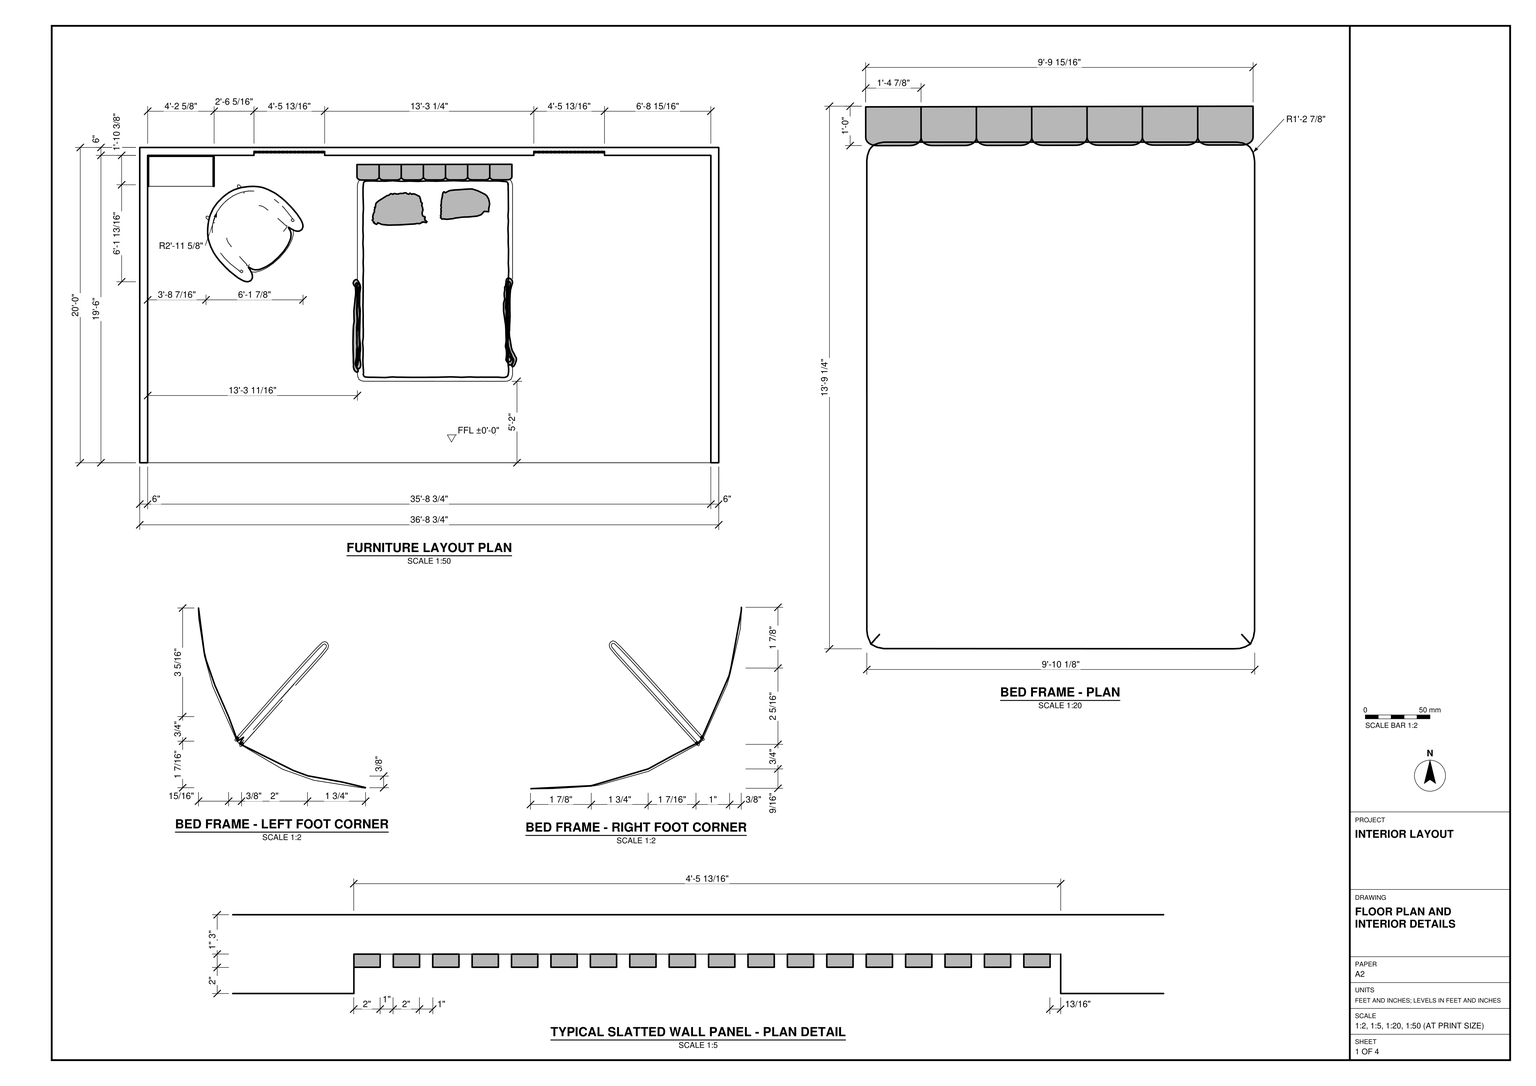
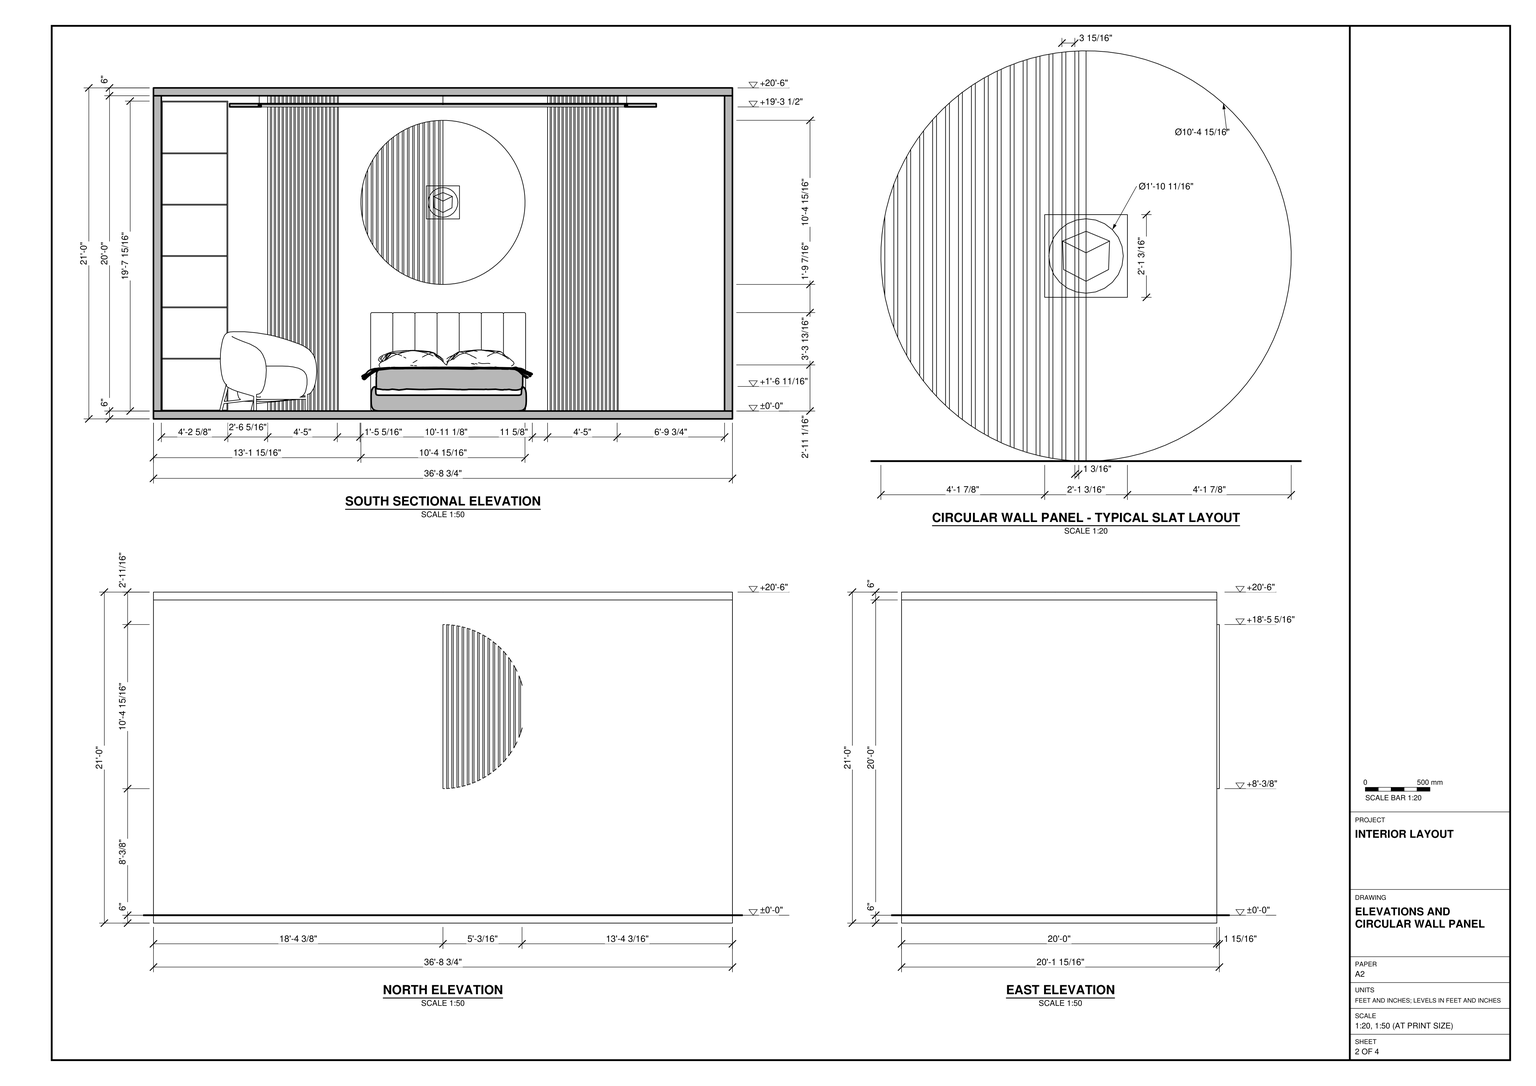
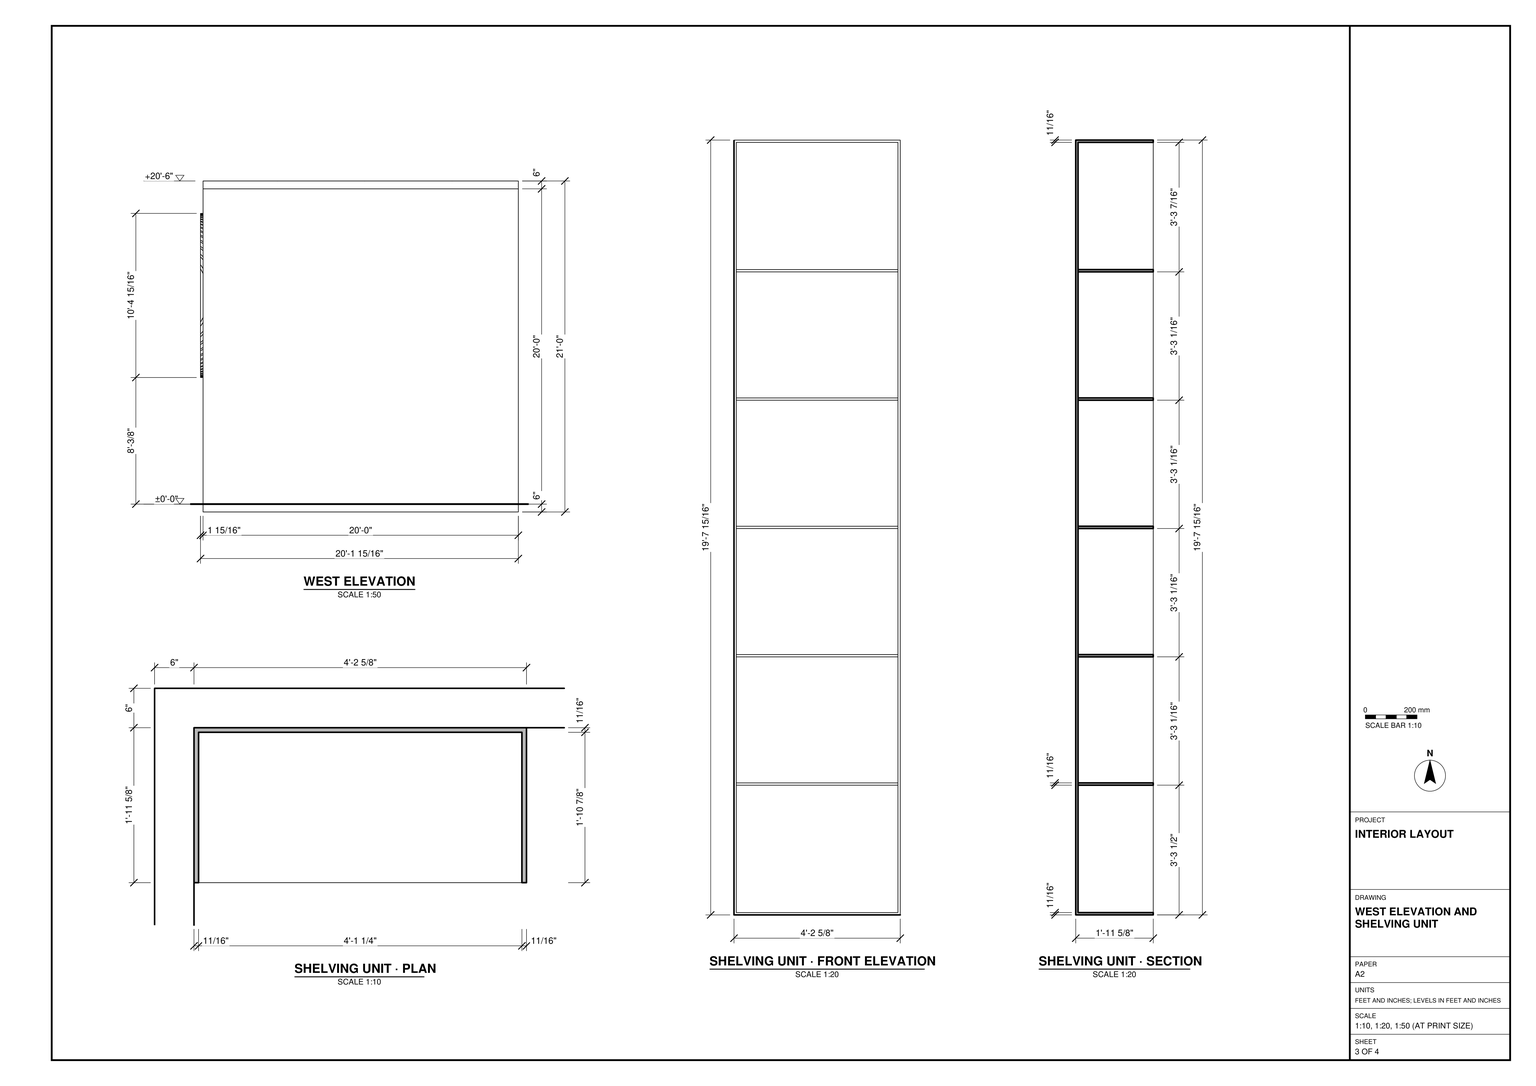
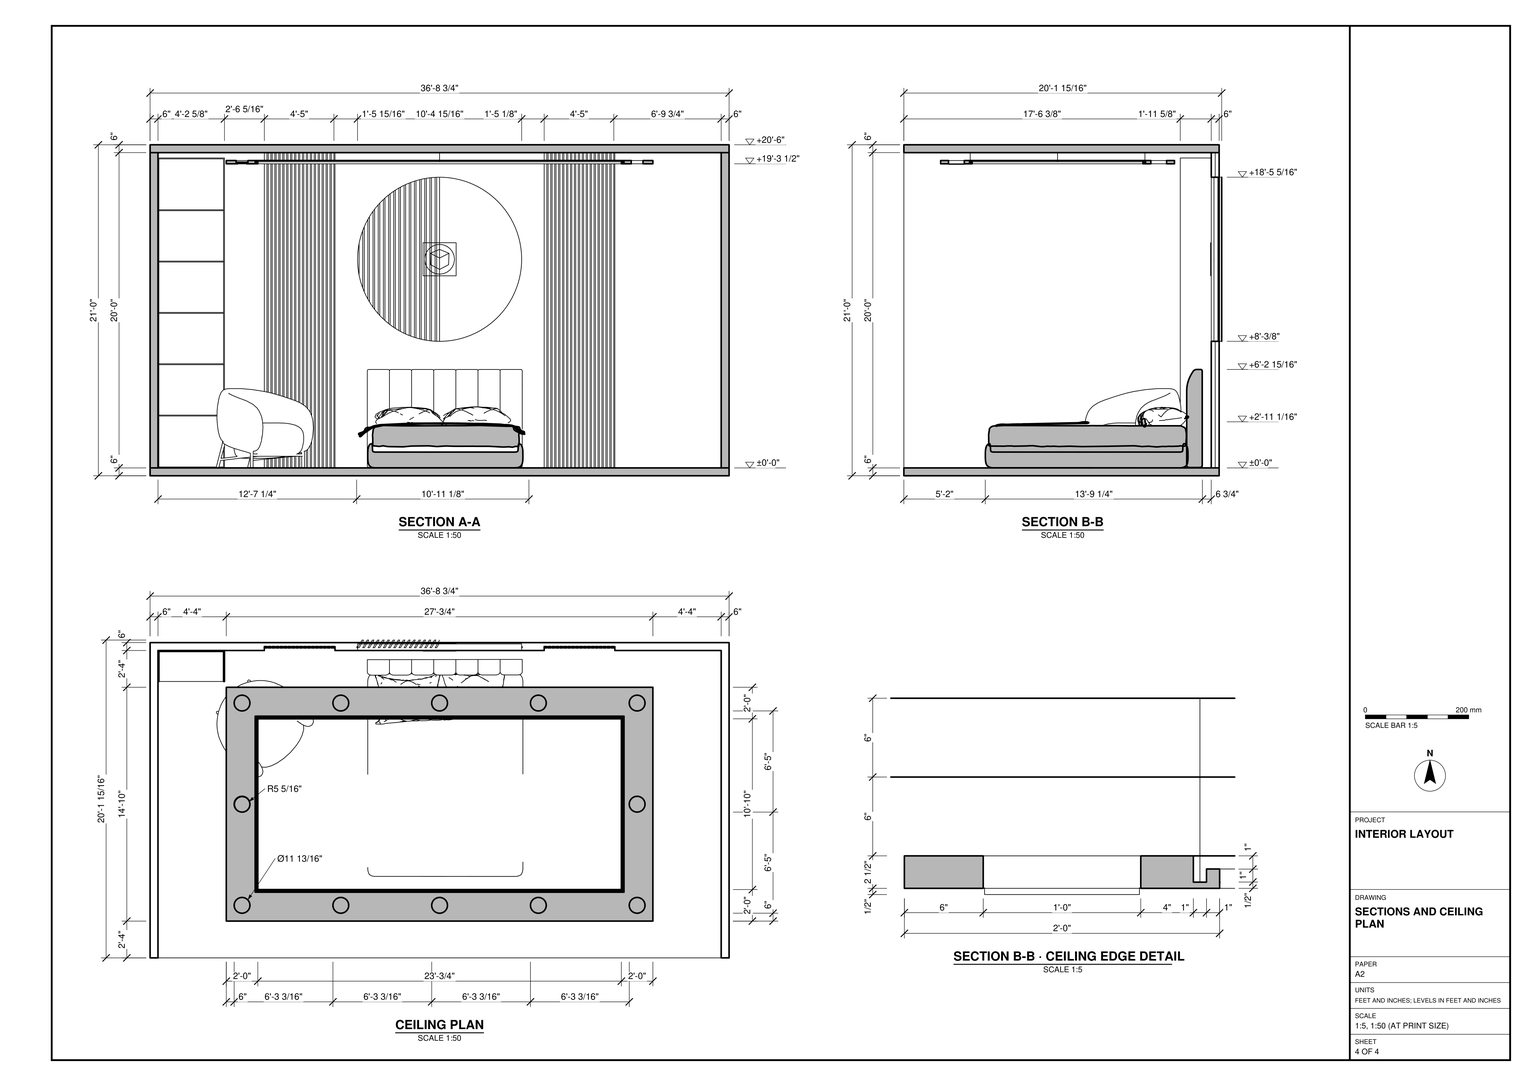
Build the bedroom interior in SketchUp from task_files/diagram_01.pdf. Work in feet and inches. Set the finished floor level to ±0'-0". The overall model, including the projecting wall detail, is 36'-8 3/4" wide, 20'-1 15/16" deep and 21'-0" high. Form the north wall and both side walls at 6" thick, leaving the south side open as drawn. Include the 6" floor and ceiling slabs, with a clear height of 20'-0" between them.

Place the bed with its segmented headboard against the north wall and its foot facing the open side. Follow the bed-frame plan for the rounded foot corners, and use the sectional elevation to set the mattress and headboard heights. Above the bed, model the circular wall panel with vertical slats on its left half and a plain field on its right. Flank the bed with the two tall rectangular slatted panels, following the spacing in the plan detail. Fit the tall open shelving unit into the northwest corner and place the armchair in front of it, angled as shown in the furniture layout.

Keep the walls and slabs separate, and make each furniture or joinery piece a separate group or component. Use components for repeated parts such as slats. Decor and loose items may be any suitable library components. Save one SketchUp model as output_files/bedroom_with_slatted_wall_panels_and_built_in_shelving.skp.

# SketchUp Ruby script. Lengths in inches.
U = 1.inch
M = Sketchup.active_model
def pt(a) = Geom::Point3d.new(a.map { |v| v * U })
def face(e, loops, mat)
  f = e.add_face(loops[0].map { |a| pt(a) })
  loops[1..].each { |l| e.add_face(l.map { |a| pt(a) }).erase! }
  f.material = f.back_material = mat if mat
  f
end
# faces: each face lists its corners as indices into pts; further lists are holes
def faces(e, pts, list, mat = nil) = list.each { |f| face(e, (f[0].is_a?(Array) ? f : [f]).map { |l| l.map { |i| pts[i] } }, mat) }
# xy, xz, yz: faces in a plane at the given z, y or x. An outline is a flat list of corners, or four numbers for a rectangle; further outlines are holes
def ring(l) = l.size == 4 ? [[l[0], l[1]], [l[2], l[1]], [l[2], l[3]], [l[0], l[3]]] : l.each_slice(2).to_a
def flat(e, list, mat, &to3) = list.each { |f| face(e, (f[0].is_a?(Array) ? f : [f]).map { |l| ring(l).map { |u, v| to3.(u, v) } }, mat) }
def xy(e, z, list, mat = nil) = flat(e, list, mat) { |x, y| [x, y, z] }
def xz(e, y, list, mat = nil) = flat(e, list, mat) { |x, z| [x, y, z] }
def yz(e, x, list, mat = nil) = flat(e, list, mat) { |y, z| [x, y, z] }
def lines(e, pts, list) = list.each { |a, b| e.add_line(pt(pts[a]), pt(pts[b])) }
# prism: a flat outline (further loops are holes) pulled along v
def prism(e, loops, v, mat = nil)
  f = face(e, loops, mat); d = Geom::Vector3d.new(v.map { |x| x * U })
  f.pushpull(f.normal.samedirection?(d) ? d.length : -d.length)
end
def box(e, o, s, mat = nil) = prism(e, [[o, [o[0] + s[0], o[1], o[2]], [o[0] + s[0], o[1] + s[1], o[2]], [o[0], o[1] + s[1], o[2]]]], [0, 0, s[2]], mat)
def at(x, y, z, deg = 0) = Geom::Transformation.translation(pt([x, y, z])) * Geom::Transformation.rotation(ORIGIN, Z_AXIS, deg.degrees)
def axes(o, x, y, z) = Geom::Transformation.new([*x, 0, *y, 0, *z, 0, *pt(o).to_a, 1])
def part(name) = M.definitions.add(name)
# library, detail: a bought-in or finely detailed component or shape, given as its bounding box
def library(name, o, s) = part(name).tap { |d| box(d.entities, o, s) }
def detail(e, o, s) = box(e.add_group.entities, o, s)
def put(e, d, t, mat = nil) = e.add_instance(d, t).tap { |i| i.material = mat if mat }
def group(e, t, mat = nil) = e.add_group.tap { |g| g.transformation = t; g.material = mat if mat }.entities
root = M.entities
M.materials.add("WALL").color = [163, 159, 147]
M.materials.add("Wood 009 27.06cm").color = [255, 255, 255]
c1 = part("Group66\#1")
p = [[0,0,0],[0,0,-7.89],[-3.85,0,-7.89],[25.04,-0.51,0],[-25.04,-0.51,0],[25.04,0.51,0],
  [25.04,0,0],[-25.04,0.51,0],[3.85,0,-7.89],[-25.04,0,0],[0,0,-12.77]]
lines(c1.entities,p,[[0,1],[1,2],[3,4],[5,6],[7,5],[1,8],[9,0],[0,6],[8,10],[4,9],[6,3],[2,10],
  [9,7]])
c2 = part("shelves")
put(c2.entities,c1,at(0,0,0))
c3 = library("BED 3",[-244.73,-59.6875,196.6875],[91.01,69.4,39.64])
c4 = library("Armchair 287 004",[-17.02,-16.23,-0.09],[34.04,32.42,30.2])
c5 = part("Group5\#1")
xy(c5.entities,0,[[-26.65,-23.47,-27.78,-20.53,-27.84,-20.33,-27.84,20.25,-27.32,21.79,-26.65,23.42]])
xy(c5.entities,5.875,[[-30.05,-12.08,-30.05,12.03,-30.37,10.43,-30.9,6.55,-31.19,2.63,-31.23,-1.29,-31.03,-5.21,-30.58,-9.11]])
p = [[-30.05,12.03,5.875],[-30.05,-12.08,5.875],[-29.89,-12.98,5.6],[-28.95,-16.79,3.98],[-27.78,-20.53,1.95],[-26.65,-23.47,0],
  [-26.65,23.42,0],[-27.32,21.79,1.15],[-28.57,18.07,3.33],[-29.59,14.28,5.09],[-31.03,-5.21,5.52],[-31.23,-1.29,5.875],
  [-31.19,2.63,5.8],[-30.9,6.55,5.3],[-30.37,10.43,4.375],[-29.59,14.28,3.03],[-28.57,18.07,1.27],[-27.84,20.25,0],
  [-27.84,-20.33,0],[-28.95,-16.79,1.92],[-29.89,-12.98,3.54],[-30.58,-9.11,4.74]]
faces(c5.entities,p,[[0,1,2,3,4,5,6,7,8,9],[10,11,12,13,14,15,16,17,18,19,20,21]])
c6 = part("Group6\#1")
xy(c6.entities,0,[[-22.72,-31.5,-22.89,-31.23,-23.9,-29.33,-23.9,29.35,-22.72,31.46]])
xy(c6.entities,5.875,[[-26.11,-24.78,-26.11,24.76,-27.3,21.85,-27.3,-21.79,-26.375,-24.2]])
p = [[-26.11,24.76,5.875],[-26.11,-24.78,5.875],[-24.74,-27.77,3.51],[-22.89,-31.23,0.29],[-22.72,-31.5,0],[-22.72,31.46,0],
  [-24.13,28.96,2.44],[-25.84,25.43,5.4],[-27.3,-21.79,5.875],[-27.3,21.85,5.875],[-25.84,25.43,3.35],[-24.13,28.96,0.39],
  [-23.9,29.35,0],[-23.9,-29.33,0],[-24.74,-27.77,1.45],[-26.375,-24.2,4.28]]
faces(c6.entities,p,[[0,1,2,3,4,5,6,7],[8,9,10,11,12,13,14,15]])
c7 = part("Group7\#1")
xy(c7.entities,0,[[-18.78,-37.4375,-19.97,-35.77,-19.97,35.8,-18.78,37.39]])
xy(c7.entities,5.875,[[-22.17,-32.38,-22.17,32.42,-22.2,32.38,-23.36,30.32,-23.36,-30.35,-22.89,-31.23]])
p = [[-18.78,-37.4375,0],[-18.78,37.39,0],[-20.06,35.67,2.22],[-22.17,32.42,5.875],[-22.17,-32.38,5.875],[-20.82,-34.57,3.53],
  [-23.36,-30.35,5.875],[-23.36,30.32,5.875],[-22.2,32.38,3.87],[-20.06,35.67,0.16],[-19.97,35.8,0],[-19.97,-35.77,0],
  [-20.82,-34.57,1.48],[-22.89,-31.23,5.06]]
faces(c7.entities,p,[[0,1,2,3,4,5],[6,7,8,9,10,11,12,13]])
c8 = part("Group8\#1")
xy(c8.entities,0,[[-14.84,-42.16,-16.03,-40.87,-16.03,40.82,-15.18,41.82,-14.84,42.17]])
xy(c8.entities,5.875,[[-18.23,-38.15,-18.23,38.125,-19.42,36.53,-19.42,-36.53,-18.55,-37.77]])
p = [[-14.84,-42.16,0],[-14.84,42.17,0],[-15.18,41.82,0.59],[-17.72,38.82,4.98],[-18.23,38.125,5.875],[-18.23,-38.15,5.875],
  [-16.08,-40.82,2.14],[-19.42,-36.53,5.875],[-19.42,36.53,5.875],[-17.72,38.82,2.93],[-16.03,40.82,0],[-16.03,-40.87,0],
  [-16.08,-40.82,0.08],[-18.55,-37.77,4.36]]
faces(c8.entities,p,[[0,1,2,3,4,5,6],[7,8,9,10,11,12,13]])
c9 = part("Group9\#1")
xy(c9.entities,0,[[-10.9,-46.125,-12.09,-44.98,-12.09,44.99,-10.9,46.08]])
xy(c9.entities,5.875,[[-14.3,-42.76,-14.3,42.74,-15.18,41.82,-15.48,41.46,-15.48,-41.46]])
p = [[-14.3,42.74,5.875],[-14.3,-42.76,5.875],[-13.42,-43.71,4.36],[-10.9,-46.125,0],[-10.9,46.08,0],[-12.47,44.65,2.7],
  [-15.48,-41.46,5.875],[-15.48,41.46,5.875],[-15.18,41.82,5.36],[-12.47,44.65,0.65],[-12.09,44.99,0],[-12.09,-44.98,0],
  [-13.42,-43.71,2.3]]
faces(c9.entities,p,[[0,1,2,3,4,5],[6,7,8,9,10,11,12]])
c10 = part("Group10\#1")
xy(c10.entities,0,[[-6.97,-49.43,-7.59,-48.96,-8.15,-48.49,-8.15,48.46,-6.97,49.42]])
xy(c10.entities,5.875,[[-10.36,-46.62,-10.36,46.59,-11.55,45.49,-11.55,-45.51,-10.59,-46.43]])
p = [[-6.97,-49.43,0],[-6.97,49.42,0],[-9.58,47.31,4.52],[-10.36,46.59,5.875],[-10.36,-46.62,5.875],[-7.59,-48.96,1.08],
  [-8.15,48.46,0],[-8.15,-48.49,0],[-10.59,-46.43,4.22],[-11.55,-45.51,5.875],[-11.55,45.49,5.875],[-9.58,47.31,2.46]]
faces(c10.entities,p,[[0,1,2,3,4,5],[6,7,8,9,10,11]])
c11 = part("Group11\#1")
xy(c11.entities,0,[[-3.03,-52.22,-4.22,-51.45,-4.22,51.41,-3.32,52.05,-3.03,52.23]])
xy(c11.entities,5.875,[[-6.42,-49.83,-6.42,49.85,-6.53,49.77,-7.61,48.9,-7.61,-48.95,-7.59,-48.96]])
p = [[-3.03,-52.22,0],[-3.03,52.23,0],[-3.32,52.05,0.51],[-6.42,49.85,5.875],[-6.42,-49.83,5.875],[-4.44,-51.3,2.45],
  [-4.22,51.41,0],[-4.22,-51.45,0],[-4.44,-51.3,0.39],[-7.59,-48.96,5.85],[-7.61,-48.95,5.875],[-7.61,48.9,5.875],
  [-6.53,49.77,4]]
faces(c11.entities,p,[[0,1,2,3,4,5],[6,7,8,9,10,11,12]])
c12 = part("Group12\#1")
xy(c12.entities,0,[[0.91,-54.6,-0.28,-53.93,-0.28,53.93,0.01,54.11,0.91,54.59]])
xy(c12.entities,5.875,[[-2.48,-52.57,-2.48,52.57,-3.32,52.05,-3.67,51.8,-3.67,-51.8]])
p = [[0.91,-54.6,0],[0.91,54.59,0],[0.01,54.11,1.55],[-2.48,52.57,5.875],[-2.48,-52.57,5.875],[-1.15,-53.44,3.57],
  [-3.67,-51.8,5.875],[-3.67,51.8,5.875],[-3.32,52.05,5.27],[-0.28,53.93,0],[-0.28,-53.93,0],[-1.15,-53.44,1.51]]
faces(c12.entities,p,[[0,1,2,3,4,5],[6,7,8,9,10,11]])
c13 = part("Group13\#1")
xy(c13.entities,0,[[4.85,-56.62,3.66,-56.04,3.66,56.05,4.85,56.6]])
xy(c13.entities,5.875,[[1.45,-54.91,1.45,54.89,0.27,54.25,0.27,-54.24]])
p = [[1.45,54.89,5.875],[1.45,-54.91,5.875],[2.27,-55.37,4.46],[4.85,-56.62,0],[4.85,56.6,0],[3.47,55.97,2.38],
  [3.66,56.05,0],[3.66,-56.04,0],[2.27,-55.37,2.41],[0.27,-54.24,5.875],[0.27,54.25,5.875],[3.47,55.97,0.32]]
faces(c13.entities,p,[[0,1,2,3,4,5],[6,7,8,9,10,11]])
c14 = part("Group14\#1")
xy(c14.entities,0,[[8.78,-58.3,7.6,-57.8125,7.6,57.8125,8.78,58.27]])
xy(c14.entities,5.875,[[5.39,-56.88,5.39,56.85,4.2,56.3,4.2,-56.31]])
p = [[8.78,-58.3,0],[8.78,58.27,0],[7.04,57.6,3.02],[5.39,56.85,5.875],[5.39,-56.88,5.875],[5.8,-57.08,5.16],
  [4.2,-56.31,5.875],[4.2,56.3,5.875],[7.04,57.6,0.96],[7.6,57.8125,0],[7.6,-57.8125,0],[5.8,-57.08,3.11]]
faces(c14.entities,p,[[0,1,2,3,4,5],[6,7,8,9,10,11]])
c15 = part("Group15\#1")
xy(c15.entities,0,[[12.72,-59.67,11.53,-59.27,11.53,59.27,12.72,59.64]])
xy(c15.entities,5.875,[[9.33,-58.52,9.33,58.48,8.14,58.02,8.14,-58.03]])
p = [[12.72,-59.67,0],[12.72,59.64,0],[10.71,59.01,3.49],[9.33,58.48,5.875],[9.33,-58.52,5.875],[9.43,-58.5625,5.69],
  [8.14,-58.03,5.875],[8.14,58.02,5.875],[10.71,59.01,1.43],[11.53,59.27,0],[11.53,-59.27,0],[9.43,-58.5625,3.63]]
faces(c15.entities,p,[[0,1,2,3,4,5],[6,7,8,9,10,11]])
c16 = part("Group16\#1")
xy(c16.entities,0,[[16.66,-60.76,15.47,-60.4375,15.47,60.43,16.66,60.72]])
xy(c16.entities,5.875,[[13.27,-59.85,13.27,59.81,12.08,59.4375,12.08,-59.45,13.15,-59.82]])
p = [[13.27,59.81,5.875],[13.27,-59.85,5.875],[16.66,-60.76,0],[16.66,60.72,0],[14.45,60.18,3.82],[12.08,-59.45,5.875],
  [12.08,59.4375,5.875],[14.45,60.18,1.76],[15.47,60.43,0],[15.47,-60.4375,0],[13.15,-59.82,4.01]]
faces(c16.entities,p,[[0,1,2,3,4],[5,6,7,8,9,10]])
c17 = part("Group17\#1")
xy(c17.entities,0,[[20.6,-61.57,19.41,-61.33,19.41,61.32,20.6,61.53]])
xy(c17.entities,5.875,[[17.2,-60.89,17.2,60.85,16.02,60.5625,16.02,-60.58,16.95,-60.83]])
p = [[20.6,-61.57,0],[20.6,61.53,0],[18.26,61.11,4.04],[17.2,60.85,5.875],[17.2,-60.89,5.875],[19.41,61.32,0],
  [19.41,-61.33,0],[16.95,-60.83,4.26],[16.02,-60.58,5.875],[16.02,60.5625,5.875],[18.26,61.11,1.98]]
faces(c17.entities,p,[[0,1,2,3,4],[5,6,7,8,9,10]])
c18 = part("Group18\#1")
xy(c18.entities,0,[[24.53,-62.125,23.35,-61.96,23.35,61.95,24.53,62.09]])
xy(c18.entities,5.875,[[21.14,-61.66,21.14,61.63,19.95,61.42,19.95,-61.44,20.79,-61.61]])
p = [[24.53,-62.125,0],[24.53,62.09,0],[22.13,61.81,4.16],[21.14,61.63,5.875],[21.14,-61.66,5.875],[19.95,-61.44,5.875],
  [19.95,61.42,5.875],[22.13,61.81,2.11],[23.35,61.95,0],[23.35,-61.96,0],[20.79,-61.61,4.42]]
faces(c18.entities,p,[[0,1,2,3,4],[5,6,7,8,9,10]])
c19 = part("Group19\#1")
xy(c19.entities,0,[[28.47,-62.42,27.28,-62.34,27.28,62.32,28.47,62.38]])
xy(c19.entities,5.875,[[25.08,-62.17,25.08,62.15,23.89,62.01,23.89,-62.04,24.68,-62.14]])
p = [[25.08,62.15,5.875],[25.08,-62.17,5.875],[28.47,-62.42,0],[28.47,62.38,0],[26.03,62.26,4.23],[23.89,-62.04,5.875],
  [23.89,62.01,5.875],[26.03,62.26,2.17],[27.28,62.32,0],[27.28,-62.34,0],[24.68,-62.14,4.5]]
faces(c19.entities,p,[[0,1,2,3,4],[5,6,7,8,9,10]])
c20 = part("Group20\#1")
xy(c20.entities,0,[[31.22,-62.46,31.23,62.45]])
xy(c20.entities,5.875,[[29.02,-62.4375,29.02,62.41,27.83,62.35,27.83,-62.375,28.6,-62.43]])
p = [[27.83,-62.375,5.875],[27.83,62.35,5.875],[29.95,62.46,2.2],[31.22,62.45,0],[31.22,-62.46,0],[28.6,-62.43,4.54],
  [29.02,62.41,5.875],[29.02,-62.4375,5.875],[31.23,-62.46,2.03],[31.23,62.45,2.03],[29.95,62.46,4.26]]
faces(c20.entities,p,[[0,1,2,3,4,5],[6,7,8,9,10]])
c21 = part("Group3\#1")
put(c21.entities,c5,at(0,0,0))
put(c21.entities,c6,at(0,0,0))
put(c21.entities,c7,at(0,0,0))
put(c21.entities,c8,at(0,0,0))
put(c21.entities,c9,at(0,0,0))
put(c21.entities,c10,at(0,0,0))
put(c21.entities,c11,at(0,0,0))
put(c21.entities,c12,at(0,0,0))
put(c21.entities,c13,at(0,0,0))
put(c21.entities,c14,at(0,0,0))
put(c21.entities,c15,at(0,0,0))
put(c21.entities,c16,at(0,0,0))
put(c21.entities,c17,at(0,0,0))
put(c21.entities,c18,at(0,0,0))
put(c21.entities,c19,at(0,0,0))
put(c21.entities,c20,at(0,0,0))
c22 = library("Mesh Light",[-0.5,-0.5,-0.1],[1,1,0.2])
c23 = part("Group25\#1")
box(c23.entities,[-26.9,-120,0],[2,240,1])
c24 = part("Group26\#1")
box(c24.entities,[-23.9,-120,0],[2,240,1])
c25 = part("Group27\#1")
box(c25.entities,[-20.9,-120,0],[2,240,1])
c26 = part("Group28\#1")
box(c26.entities,[-17.9,-120,0],[2,240,1])
c27 = part("Group29\#1")
box(c27.entities,[-14.9,-120,0],[2,240,1])
c28 = part("Group30\#1")
box(c28.entities,[-11.9,-120,0],[2,240,1])
c29 = part("Group31\#1")
box(c29.entities,[-8.9,-120,0],[2,240,1])
c30 = part("Group32\#1")
box(c30.entities,[-5.9,-120,0],[2,240,1])
c31 = part("Group33\#1")
box(c31.entities,[-2.9,-120,0],[2,240,1])
c32 = part("Group34\#1")
box(c32.entities,[0.1,-120,0],[2,240,1])
c33 = part("Group35\#1")
box(c33.entities,[3.1,-120,0],[2,240,1])
c34 = part("Group36\#1")
box(c34.entities,[6.1,-120,0],[2,240,1])
c35 = part("Group37\#1")
box(c35.entities,[9.1,-120,0],[2,240,1])
c36 = part("Group38\#1")
box(c36.entities,[12.1,-120,0],[2,240,1])
c37 = part("Group39\#1")
box(c37.entities,[15.1,-120,0],[2,240,1])
c38 = part("Group40\#1")
box(c38.entities,[18.1,-120,0],[2,240,1])
c39 = part("Group41\#1")
box(c39.entities,[21.1,-120,0],[2,240,1])
c40 = part("Group42\#1")
box(c40.entities,[24.1,-120,0],[2,240,1])
c41 = part("Group23\#1")
put(c41.entities,c23,at(0,0,0))
put(c41.entities,c24,at(0,0,0))
put(c41.entities,c25,at(0,0,0))
put(c41.entities,c26,at(0,0,0))
put(c41.entities,c27,at(0,0,0))
put(c41.entities,c28,at(0,0,0))
put(c41.entities,c29,at(0,0,0))
put(c41.entities,c30,at(0,0,0))
put(c41.entities,c31,at(0,0,0))
put(c41.entities,c32,at(0,0,0))
put(c41.entities,c33,at(0,0,0))
put(c41.entities,c34,at(0,0,0))
put(c41.entities,c35,at(0,0,0))
put(c41.entities,c36,at(0,0,0))
put(c41.entities,c37,at(0,0,0))
put(c41.entities,c38,at(0,0,0))
put(c41.entities,c39,at(0,0,0))
put(c41.entities,c40,at(0,0,0))
c42 = part("Group44\#1")
box(c42.entities,[-26.9,-120,0],[2,240,1])
c43 = part("Group45\#1")
box(c43.entities,[-23.9,-120,0],[2,240,1])
c44 = part("Group46\#1")
box(c44.entities,[-20.9,-120,0],[2,240,1])
c45 = part("Group47\#1")
box(c45.entities,[-17.9,-120,0],[2,240,1])
c46 = part("Group48\#1")
box(c46.entities,[-14.9,-120,0],[2,240,1])
c47 = part("Group49\#1")
box(c47.entities,[-11.9,-120,0],[2,240,1])
c48 = part("Group50\#1")
box(c48.entities,[-8.9,-120,0],[2,240,1])
c49 = part("Group51\#1")
box(c49.entities,[-5.9,-120,0],[2,240,1])
c50 = part("Group52\#1")
box(c50.entities,[-2.9,-120,0],[2,240,1])
c51 = part("Group53\#1")
box(c51.entities,[0.1,-120,0],[2,240,1])
c52 = part("Group54\#1")
box(c52.entities,[3.1,-120,0],[2,240,1])
c53 = part("Group55\#1")
box(c53.entities,[6.1,-120,0],[2,240,1])
c54 = part("Group56\#1")
box(c54.entities,[9.1,-120,0],[2,240,1])
c55 = part("Group57\#1")
box(c55.entities,[12.1,-120,0],[2,240,1])
c56 = part("Group58\#1")
box(c56.entities,[15.1,-120,0],[2,240,1])
c57 = part("Group59\#1")
box(c57.entities,[18.1,-120,0],[2,240,1])
c58 = part("Group60\#1")
box(c58.entities,[21.1,-120,0],[2,240,1])
c59 = part("Group61\#1")
box(c59.entities,[24.1,-120,0],[2,240,1])
c60 = part("Group42\#2")
put(c60.entities,c42,at(0,0,0))
put(c60.entities,c43,at(0,0,0))
put(c60.entities,c44,at(0,0,0))
put(c60.entities,c45,at(0,0,0))
put(c60.entities,c46,at(0,0,0))
put(c60.entities,c47,at(0,0,0))
put(c60.entities,c48,at(0,0,0))
put(c60.entities,c49,at(0,0,0))
put(c60.entities,c50,at(0,0,0))
put(c60.entities,c51,at(0,0,0))
put(c60.entities,c52,at(0,0,0))
put(c60.entities,c53,at(0,0,0))
put(c60.entities,c54,at(0,0,0))
put(c60.entities,c55,at(0,0,0))
put(c60.entities,c56,at(0,0,0))
put(c60.entities,c57,at(0,0,0))
put(c60.entities,c58,at(0,0,0))
put(c60.entities,c59,at(0,0,0))
c61 = part("Group")
box(c61.entities,[0,0,0],[440.75,240,6])
c62 = part("Group\#5")
box(c62.entities,[0,0,0],[50.07,23.29,0.71])
c63 = library("Group\#6",[0,0,-0.94],[324.76,178,71.14])
put(root,c2,axes([31.3125,232.8,234.75],[0.9831,0,0],[0,-0.9831,0],[0,0,0.9831]))
put(root,c2,axes([31.3125,232.8,195.31],[0.9831,0,0],[0,-0.9831,0],[0,0,0.9831]))
put(root,c2,axes([31.3125,232.8,155.24],[0.9831,0,0],[0,-0.9831,0],[0,0,0.9831]))
put(root,c2,axes([31.3125,232.8,113.59],[0.9831,0,0],[0,-0.9831,0],[0,0,0.9831]))
put(root,c2,axes([31.3125,232.8,75.61],[0.9831,0,0],[0,-0.9831,0],[0,0,0.9831]))
put(root,c2,axes([31.3125,232.8,36.54],[0.9831,0,0],[0,-0.9831,0],[0,0,0.9831]))
put(root,c3,axes([270.05,-228.54,-371.74],[0,-1.89,0],[1.89,0,0],[0,0,1.89]))
put(root,c4,axes([83.28,178.77,0.18],[1.41421,1.41421,0],[-1.41421,1.41421,0],[0,0,2]))
g1 = group(root,at(0,0,0))
xy(g1,0,[[0,0,0,240,440.75,240,440.75,0,434.75,0,434.75,234,353.8,234,353.8,237,299.99,237,299.99,234,140.76,234,140.76,237,86.95,237,86.95,234,6,234,6,0]])
xy(g1,240,[[0,0,6,0,6,234,86.95,234,86.95,237,140.76,237,140.76,234,299.99,234,299.99,237,353.8,237,353.8,234,434.75,234,434.75,0,440.75,0,440.75,240,0,240]])
xz(g1,0,[[0,0,6,240],[434.75,0,440.75,240]])
xz(g1,234,[[6,0,86.95,240],[[140.76,0,299.99,240],[221.66,96.36,220.375,96.37,217.74,96.4,213.82,96.69,209.93,97.22,206.09,98,202.3,99.02,198.58,100.27,194.94,101.76,191.41,103.47,187.99,105.39,184.7,107.53,181.55,109.875,178.55,112.41,175.72,115.125,173.0625,118.02,170.59,121.07,168.32,124.27,166.25,127.61,164.4,131.06,162.77,134.63,161.36,138.3,160.1875,142.05,159.25,145.86,158.56,149.72,158.11,153.62,157.91,157.54,157.95,161.47,158.24,165.38,158.77,169.27,159.55,173.12,160.57,176.91,161.82,180.625,163.3,184.26,165.01,187.79,166.94,191.21,169.08,194.5,171.42,197.65,173.96,200.65,176.67,203.48,179.5625,206.14,182.62,208.61,185.82,210.88,189.15,212.95,192.61,214.8,196.18,216.44,199.85,217.84,203.59,219.01,207.41,219.95,211.27,220.64,215.17,221.09,219.09,221.3,220.375,221.28,223.01,221.25,226.93,220.96,230.82,220.43,234.66,219.65,238.45,218.64,242.17,217.38,245.81,215.9,249.34,214.1875,252.76,212.26,256.05,210.12,259.2,207.78,262.2,205.25,265.03,202.53,267.6875,199.64,270.16,196.59,272.43,193.39,274.5,190.05,276.35,186.59,277.98,183.02,279.39,179.36,280.5625,175.61,281.5,171.8,282.19,167.93,282.64,164.03,282.84,160.11,282.8,156.1875,282.51,152.27,281.98,148.39,281.2,144.54,280.18,140.75,278.93,137.03,277.45,133.39,275.74,129.86,273.81,126.44,271.67,123.15,269.33,120,266.79,117,264.08,114.17,261.1875,111.51,258.13,109.05,254.93,106.77,251.6,104.71,248.14,102.85,244.57,101.22,240.9,99.8125,237.16,98.64,233.34,97.71,229.48,97.01,225.58,96.5625]],[353.8,0,434.75,240]])
xz(g1,239,[[221.66,96.36,225.58,96.5625,229.48,97.01,233.34,97.71,237.16,98.64,240.9,99.8125,244.57,101.22,248.14,102.85,251.6,104.71,254.93,106.77,258.13,109.05,261.1875,111.51,264.08,114.17,266.79,117,269.33,120,271.67,123.15,273.81,126.44,275.74,129.86,277.45,133.39,278.93,137.03,280.18,140.75,281.2,144.54,281.98,148.39,282.51,152.27,282.8,156.1875,282.84,160.11,282.64,164.03,282.19,167.93,281.5,171.8,280.5625,175.61,279.39,179.36,277.98,183.02,276.35,186.59,274.5,190.05,272.43,193.39,270.16,196.59,267.6875,199.64,265.03,202.53,262.2,205.25,259.2,207.78,256.05,210.12,252.76,212.26,249.34,214.1875,245.81,215.9,242.17,217.38,238.45,218.64,234.66,219.65,230.82,220.43,226.93,220.96,223.01,221.25,220.375,221.28,220.375,96.37]],"WALL")
xz(g1,240,[[0,0,440.75,240]])
yz(g1,0,[[0,0,240,240]])
yz(g1,6,[[0,0,234,240]])
yz(g1,86.95,[[234,0,237,240]])
yz(g1,140.76,[[234,0,237,240]])
yz(g1,299.99,[[234,0,237,240]])
yz(g1,353.8,[[234,0,237,240]])
yz(g1,434.75,[[0,0,234,240]])
yz(g1,440.75,[[0,0,240,240]])
put(g1,c21,axes([189.14,241.9375,158.83],[1,0,0],[0,0,1],[0,-1,0]))
g2 = group(g1,at(157.91,234,96.36))
p = [[55.92,0,0.33],[59.83,0,0.04],[59.83,5,0.04],[55.92,5,0.33],[62.47,0,0.01],[63.76,0,0],
  [63.76,5,0],[62.47,5,0.01],[67.68,0,0.2],[67.68,5,0.2],[71.57,0,0.65],[71.57,5,0.65],
  [52.03,0,0.87],[52.03,5,0.87],[75.4375,0,1.35],[75.4375,5,1.35],[48.18,0,1.64],[48.18,5,1.64],
  [79.25,0,2.28],[79.25,5,2.28],[44.39,0,2.66],[44.39,5,2.66],[83,0,3.46],[83,5,3.46],
  [40.67,0,3.91],[40.67,5,3.91],[86.66,0,4.86],[86.66,5,4.86],[37.04,0,5.4],[37.04,5,5.4],
  [90.23,0,6.49],[90.23,5,6.49],[33.5,0,7.11],[33.5,5,7.11],[93.69,0,8.35],[93.69,5,8.35],
  [30.08,0,9.04],[30.08,5,9.04],[97.03,0,10.41],[97.03,5,10.41],[26.79,0,11.17],[26.79,5,11.17],
  [100.23,0,12.6875],[100.23,5,12.6875],[23.64,0,13.52],[23.64,5,13.52],[103.28,0,15.16],[103.28,5,15.16],
  [20.64,0,16.05],[20.64,5,16.05],[106.17,0,17.8125],[106.17,5,17.8125],[17.8125,0,18.77],[17.8125,5,18.77],
  [108.89,0,20.64],[108.89,5,20.64],[15.16,0,21.66],[15.16,5,21.66],[111.42,0,23.64],[111.42,5,23.64],
  [12.6875,0,24.71],[12.6875,5,24.71],[113.76,0,26.79],[113.76,5,26.79],[10.41,0,27.91],[10.41,5,27.91],
  [115.9,0,30.08],[115.9,5,30.08],[8.35,0,31.25],[8.35,5,31.25],[117.83,0,33.5],[117.83,5,33.5],
  [6.49,0,34.71],[6.49,5,34.71],[119.54,0,37.04],[119.54,5,37.04],[4.86,0,38.28],[4.86,5,38.28],
  [121.02,0,40.67],[121.02,5,40.67],[3.46,0,41.94],[3.46,5,41.94],[122.28,0,44.39],[122.28,5,44.39],
  [2.28,0,45.6875],[2.28,5,45.6875],[123.29,0,48.18],[123.29,5,48.18],[1.35,0,49.5],[1.35,5,49.5],
  [124.07,0,52.03],[124.07,5,52.03],[0.65,0,53.36],[0.65,5,53.36],[124.61,0,55.92],[124.61,5,55.92],
  [0.2,0,57.26],[0.2,5,57.26],[124.89,0,59.83],[124.89,5,59.83],[0,0,61.18],[0,5,61.18],
  [124.9375,0,63.76],[124.9375,5,63.76],[0.04,0,65.11],[0.04,5,65.11],[124.73,0,67.68],[124.73,5,67.68],
  [0.33,0,69.02],[0.33,5,69.02],[124.28,0,71.57],[124.28,5,71.57],[0.87,0,72.91],[0.87,5,72.91],
  [123.59,0,75.4375],[123.59,5,75.4375],[1.64,0,76.76],[1.64,5,76.76],[122.65,0,79.25],[122.65,5,79.25],
  [2.66,0,80.55],[2.66,5,80.55],[121.48,0,83],[121.48,5,83],[3.91,0,84.27],[3.91,5,84.27],
  [120.08,0,86.66],[120.08,5,86.66],[5.4,0,87.9],[5.4,5,87.9],[118.44,0,90.23],[118.44,5,90.23],
  [7.11,0,91.44],[7.11,5,91.44],[116.59,0,93.69],[116.59,5,93.69],[9.04,0,94.85],[9.04,5,94.85],
  [114.52,0,97.03],[114.52,5,97.03],[11.17,0,98.15],[11.17,5,98.15],[112.25,0,100.23],[112.25,5,100.23],
  [13.52,0,101.3],[13.52,5,101.3],[109.78,0,103.28],[109.78,5,103.28],[16.05,0,104.29],[16.05,5,104.29],
  [107.125,0,106.17],[107.125,5,106.17],[18.77,0,107.125],[18.77,5,107.125],[104.29,0,108.89],[104.29,5,108.89],
  [21.66,0,109.78],[21.66,5,109.78],[101.3,0,111.42],[101.3,5,111.42],[24.71,0,112.25],[24.71,5,112.25],
  [98.15,0,113.76],[98.15,5,113.76],[27.91,0,114.52],[27.91,5,114.52],[94.85,0,115.9],[94.85,5,115.9],
  [31.25,0,116.59],[31.25,5,116.59],[91.44,0,117.83],[91.44,5,117.83],[34.71,0,118.44],[34.71,5,118.44],
  [87.9,0,119.54],[87.9,5,119.54],[38.28,0,120.08],[38.28,5,120.08],[84.27,0,121.02],[84.27,5,121.02],
  [41.94,0,121.48],[41.94,5,121.48],[80.55,0,122.28],[80.55,5,122.28],[45.6875,0,122.65],[45.6875,5,122.65],
  [76.76,0,123.29],[76.76,5,123.29],[49.5,0,123.59],[49.5,5,123.59],[72.91,0,124.07],[72.91,5,124.07],
  [53.36,0,124.28],[53.36,5,124.28],[69.02,0,124.61],[69.02,5,124.61],[57.26,0,124.73],[57.26,5,124.73],
  [65.11,0,124.89],[65.11,5,124.89],[61.18,0,124.9375],[61.18,5,124.9375],[62.47,0,124.92],[62.47,5,124.92]]
faces(g2,p,[[0,1,2,3],[1,4,5,6,7,2],[5,8,9,6],[8,10,11,9],[12,0,3,13],[10,14,15,11],[16,12,13,17],[14,18,19,15],
  [20,16,17,21],[18,22,23,19],[24,20,21,25],[22,26,27,23],[28,24,25,29],[26,30,31,27],[32,28,29,33],[30,34,35,31],
  [36,32,33,37],[34,38,39,35],[40,36,37,41],[38,42,43,39],[44,40,41,45],[42,46,47,43],[48,44,45,49],[46,50,51,47],
  [52,48,49,53],[50,54,55,51],[56,52,53,57],[54,58,59,55],[60,56,57,61],[58,62,63,59],[64,60,61,65],[62,66,67,63],
  [68,64,65,69],[66,70,71,67],[72,68,69,73],[70,74,75,71],[76,72,73,77],[74,78,79,75],[80,76,77,81],[78,82,83,79],
  [84,80,81,85],[82,86,87,83],[88,84,85,89],[86,90,91,87],[92,88,89,93],[90,94,95,91],[96,92,93,97],[94,98,99,95],
  [100,96,97,101],[98,102,103,99],[104,100,101,105],[102,106,107,103],[108,104,105,109],[106,110,111,107],[112,108,109,113],[110,114,115,111],
  [116,112,113,117],[114,118,119,115],[120,116,117,121],[118,122,123,119],[124,120,121,125],[122,126,127,123],[128,124,125,129],[126,130,131,127],
  [132,128,129,133],[130,134,135,131],[136,132,133,137],[134,138,139,135],[140,136,137,141],[138,142,143,139],[144,140,141,145],[142,146,147,143],
  [148,144,145,149],[146,150,151,147],[152,148,149,153],[150,154,155,151],[156,152,153,157],[154,158,159,155],[160,156,157,161],[158,162,163,159],
  [164,160,161,165],[162,166,167,163],[168,164,165,169],[166,170,171,167],[172,168,169,173],[170,174,175,171],[176,172,173,177],[174,178,179,175],
  [180,176,177,181],[178,182,183,179],[184,180,181,185],[182,186,187,183],[188,184,185,189],[186,190,191,187],[192,188,189,193],[190,194,195,191],
  [196,192,193,197],[194,198,199,195],[200,196,197,201],[198,202,200,201,203,199]])
put(g2,c22,axes([62.47,2.5,62.47],[125.9373,0,0],[0,6,0],[0,0,125.9373]))
put(g1,c41,axes([113.85,237,120],[1,0,0],[0,0,1],[0,-1,0]),"Wood 009 27.06cm")
put(g1,c60,axes([326.9,237,120],[1,0,0],[0,0,1],[0,-1,0]),"Wood 009 27.06cm")
put(root,c61,at(0,0,-6))
put(root,c61,at(0,0,240))
put(root,c62,axes([6.7,210.41,78.57],[0.9831,0,0],[0,0.9831,0],[0,0,0.9831]))
g3 = group(root,at(6.7,210.41,117.65))
box(g3,[0,0,0],[49.23,22.9,0.7])
put(root,c62,axes([6.7,210.41,156.73],[0.9831,0,0],[0,0.9831,0],[0,0,0.9831]))
put(root,c62,axes([6.7,210.41,195.81],[0.9831,0,0],[0,0.9831,0],[0,0,0.9831]))
put(root,c62,axes([6.7,210.41,39.49],[0.9831,0,0],[0,0.9831,0],[0,0,0.9831]))
g4 = group(root,at(6,210.41,0))
xy(g4,0,[[0,0,50.62,23.59]])
xy(g4,0.7,[[0.7,0,49.92,22.9]])
xy(g4,235.25,[[0.7,0,49.92,22.9]])
xy(g4,235.94,[[0,0,50.62,23.59]])
xz(g4,0,[[[0,0,50.62,235.94],[0.7,0.7,49.92,235.25]]])
xz(g4,22.9,[[0.7,0.7,49.92,235.25]])
xz(g4,23.59,[[0,0,50.62,235.94]])
yz(g4,0,[[0,0,23.59,235.94]])
yz(g4,0.7,[[0,0.7,22.9,235.25]])
yz(g4,49.92,[[0,0.7,22.9,235.25]])
yz(g4,50.62,[[0,0,23.59,235.94]])
put(root,c63,at(57.99,28,232))
